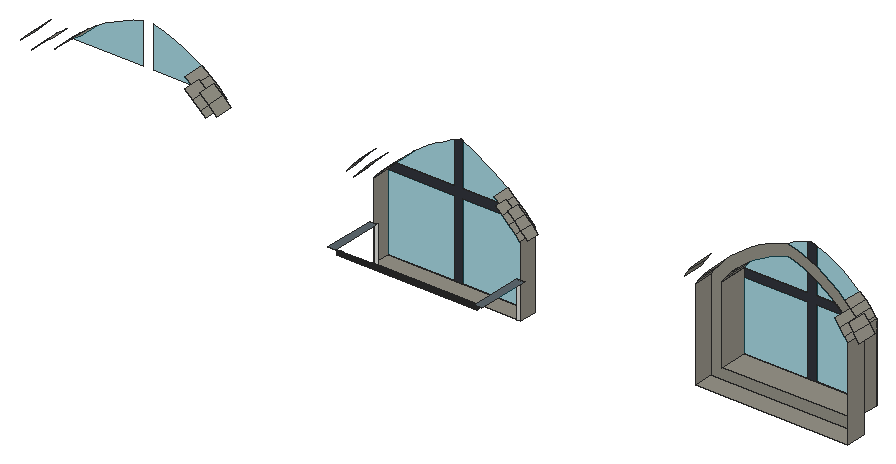
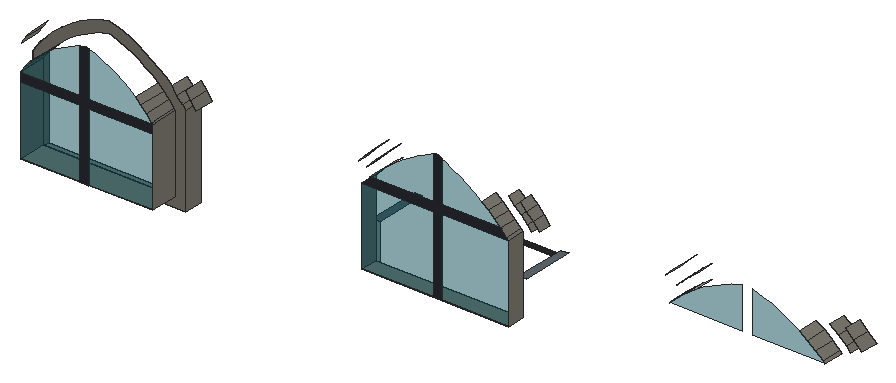
# SketchUp Ruby script. Lengths in inches.
U = 1.inch
M = Sketchup.active_model
def pt(a) = Geom::Point3d.new(a.map { |v| v * U })
def face(e, loops, mat)
  f = e.add_face(loops[0].map { |a| pt(a) })
  loops[1..].each { |l| e.add_face(l.map { |a| pt(a) }).erase! }
  f.material = f.back_material = mat if mat
  f
end
# faces: each face lists its corners as indices into pts; further lists are holes
def faces(e, pts, list, mat = nil) = list.each { |f| face(e, (f[0].is_a?(Array) ? f : [f]).map { |l| l.map { |i| pts[i] } }, mat) }
# xy, xz, yz: faces in a plane at the given z, y or x. An outline is a flat list of corners, or four numbers for a rectangle; further outlines are holes
def ring(l) = l.size == 4 ? [[l[0], l[1]], [l[2], l[1]], [l[2], l[3]], [l[0], l[3]]] : l.each_slice(2).to_a
def flat(e, list, mat, &to3) = list.each { |f| face(e, (f[0].is_a?(Array) ? f : [f]).map { |l| ring(l).map { |u, v| to3.(u, v) } }, mat) }
def xy(e, z, list, mat = nil) = flat(e, list, mat) { |x, y| [x, y, z] }
def xz(e, y, list, mat = nil) = flat(e, list, mat) { |x, z| [x, y, z] }
def yz(e, x, list, mat = nil) = flat(e, list, mat) { |y, z| [x, y, z] }
def lines(e, pts, list) = list.each { |a, b| e.add_line(pt(pts[a]), pt(pts[b])) }
# prism: a flat outline (further loops are holes) pulled along v
def prism(e, loops, v, mat = nil)
  f = face(e, loops, mat); d = Geom::Vector3d.new(v.map { |x| x * U })
  f.pushpull(f.normal.samedirection?(d) ? d.length : -d.length)
end
def box(e, o, s, mat = nil) = prism(e, [[o, [o[0] + s[0], o[1], o[2]], [o[0] + s[0], o[1] + s[1], o[2]], [o[0], o[1] + s[1], o[2]]]], [0, 0, s[2]], mat)
def at(x, y, z, deg = 0) = Geom::Transformation.translation(pt([x, y, z])) * Geom::Transformation.rotation(ORIGIN, Z_AXIS, deg.degrees)
def axes(o, x, y, z) = Geom::Transformation.new([*x, 0, *y, 0, *z, 0, *pt(o).to_a, 1])
def part(name) = M.definitions.add(name)
# library, detail: a bought-in or finely detailed component or shape, given as its bounding box
def library(name, o, s) = part(name).tap { |d| box(d.entities, o, s) }
def detail(e, o, s) = box(e.add_group.entities, o, s)
def put(e, d, t, mat = nil) = e.add_instance(d, t).tap { |i| i.material = mat if mat }
def group(e, t, mat = nil) = e.add_group.tap { |g| g.transformation = t; g.material = mat if mat }.entities
root = M.entities
M.materials.add("[Color M07]").color = [58, 58, 58]
M.materials.add("[Formica Graystone]").color = [149, 146, 135]
M.materials.add("[Formica Laminate Dark]").color = [50, 53, 60]
M.materials.add("[Formica Speckled Grey]").color = [94, 105, 111]
M.materials.add("[Translucent Glass Tinted]").color = [4, 106, 127]
M.materials["[Translucent Glass Tinted]"].alpha = 0.48
xy(root,454.81,[[376.06,148.68,450.98,158.3]],"[Formica Graystone]")
xy(root,456.09,[[222.16,144.04,294.2,152.54]],"[Formica Graystone]")
xy(root,459.9,[[381.16,158.3,445.88,172.24]],"[Formica Graystone]")
xy(root,471.52,[[287.21,119.22,287.43,119.22,287.63,119.28,287.8125,119.39,287.96,119.54,288.07,119.72,288.12,119.93,288.12,120.14,288.06,120.35,287.95,120.53,287.8,120.68,287.61,120.78,287.41,120.83,287.2,120.83,286.99,120.77,286.81,120.67,286.66,120.51,286.56,120.33,286.5,120.125,286.51,119.91,286.5625,119.71,286.67,119.52,286.82,119.375,287.01,119.27]])
xy(root,471.61,[[269.03,119.22,269.24,119.22,269.44,119.28,269.625,119.39,269.77,119.54,269.88,119.72,269.93,119.93,269.93,120.14,269.87,120.35,269.76,120.53,269.67,120.62,268.58,120.62,268.47,120.51,268.37,120.33,268.32,120.125,268.32,119.91,268.375,119.71,268.48,119.52,268.64,119.375,268.82,119.27],[268.58,120.62,269.67,120.62,269.61,120.68,269.43,120.78,269.22,120.83,269.01,120.83,268.8,120.77,268.62,120.67]])
xy(root,471.82,[[251.53,119.22,251.74,119.22,251.94,119.28,252.125,119.39,252.27,119.54,252.38,119.72,252.43,119.93,252.43,120.14,252.37,120.35,252.26,120.53,252.11,120.68,252.06,120.71,251.19,120.71,251.12,120.67,250.97,120.51,250.87,120.33,250.82,120.125,250.82,119.91,250.875,119.71,250.98,119.52,251.14,119.375,251.32,119.27],[254.4,119.22,254.61,119.22,254.82,119.28,255,119.39,255.15,119.54,255.25,119.72,255.31,119.93,255.3,120.14,255.25,120.35,255.14,120.53,254.99,120.68,254.93,120.71,254.07,120.71,254,120.67,253.85,120.51,253.75,120.33,253.69,120.125,253.69,119.91,253.75,119.71,253.86,119.52,254.01,119.375,254.2,119.27],[257.53,119.22,257.74,119.22,257.94,119.28,258.125,119.39,258.27,119.54,258.38,119.72,258.43,119.93,258.43,120.14,258.37,120.35,258.26,120.53,258.11,120.68,258.06,120.71,257.19,120.71,257.12,120.67,256.97,120.51,256.87,120.33,256.82,120.125,256.82,119.91,256.875,119.71,256.98,119.52,257.14,119.375,257.32,119.27],[266.15,119.22,266.36,119.22,266.57,119.28,266.75,119.39,266.9,119.54,267,119.72,267.06,119.93,267.05,120.14,267,120.35,266.89,120.53,266.74,120.68,266.68,120.71,265.82,120.71,265.75,120.67,265.6,120.51,265.5,120.33,265.44,120.125,265.44,119.91,265.5,119.71,265.61,119.52,265.76,119.375,265.95,119.27],[251.19,120.71,252.06,120.71,251.93,120.78,251.72,120.83,251.51,120.83,251.3,120.77],
  [254.07,120.71,254.93,120.71,254.8,120.78,254.6,120.83,254.38,120.83,254.18,120.77],[257.19,120.71,258.06,120.71,257.93,120.78,257.72,120.83,257.51,120.83,257.3,120.77],[265.82,120.71,266.68,120.71,266.55,120.78,266.35,120.83,266.13,120.83,265.93,120.77]])
xy(root,471.83,[[274.78,119.22,274.99,119.22,275.19,119.28,275.375,119.39,275.52,119.54,275.63,119.72,275.68,119.93,275.68,120.14,275.62,120.35,275.51,120.53,275.36,120.68,275.18,120.78,274.97,120.83,274.76,120.83,274.55,120.77,274.37,120.67,274.22,120.51,274.12,120.33,274.07,120.125,274.07,119.91,274.125,119.71,274.23,119.52,274.39,119.375,274.57,119.27]])
xy(root,472.05,[[231.4,119.22,231.61,119.22,231.82,119.28,232,119.39,232.15,119.54,232.25,119.72,232.31,119.93,232.3,120.14,232.25,120.35,232.14,120.53,231.99,120.68,231.88,120.74,231.12,120.74,231,120.67,230.85,120.51,230.75,120.33,230.69,120.125,230.69,119.91,230.75,119.71,230.86,119.52,231.01,119.375,231.2,119.27],[237.15,119.22,237.36,119.22,237.57,119.28,237.75,119.39,237.9,119.54,238,119.72,238.06,119.93,238.05,120.14,238,120.35,237.89,120.53,237.74,120.68,237.63,120.74,236.87,120.74,236.75,120.67,236.6,120.51,236.5,120.33,236.44,120.125,236.44,119.91,236.5,119.71,236.61,119.52,236.76,119.375,236.95,119.27],[248.65,119.22,248.86,119.22,249.07,119.28,249.25,119.39,249.4,119.54,249.5,119.72,249.56,119.93,249.55,120.14,249.5,120.35,249.39,120.53,249.24,120.68,249.13,120.74,248.37,120.74,248.25,120.67,248.1,120.51,248,120.33,247.94,120.125,247.94,119.91,248,119.71,248.11,119.52,248.26,119.375,248.45,119.27],[271.9,119.22,272.11,119.22,272.32,119.28,272.5,119.39,272.65,119.54,272.75,119.72,272.81,119.93,272.8,120.14,272.75,120.35,272.64,120.53,272.49,120.68,272.38,120.74,271.62,120.74,271.5,120.67,271.35,120.51,271.25,120.33,271.19,120.125,271.19,119.91,271.25,119.71,271.36,119.52,271.51,119.375,271.7,119.27],[290.78,119.22,290.99,119.22,291.19,119.28,291.375,119.39,291.52,119.54,291.63,119.72,291.68,119.93,291.68,120.14,291.62,120.35,291.51,120.53,291.36,120.68,291.25,120.74,290.49,120.74,290.37,120.67,290.22,120.51,290.12,120.33,290.07,120.125,290.07,119.91,290.125,119.71,290.23,119.52,290.39,119.375,290.57,119.27],
  [231.12,120.74,231.88,120.74,231.8,120.78,231.6,120.83,231.38,120.83,231.18,120.77],[236.87,120.74,237.63,120.74,237.55,120.78,237.35,120.83,237.13,120.83,236.93,120.77],[248.37,120.74,249.13,120.74,249.05,120.78,248.85,120.83,248.63,120.83,248.43,120.77],[271.62,120.74,272.38,120.74,272.3,120.78,272.1,120.83,271.88,120.83,271.68,120.77],[290.49,120.74,291.25,120.74,291.18,120.78,290.97,120.83,290.76,120.83,290.55,120.77]])
xy(root,472.27,[[225.65,119.22,225.86,119.22,226.07,119.28,226.25,119.39,226.4,119.54,226.5,119.72,226.56,119.93,226.55,120.14,226.5,120.35,226.39,120.53,226.24,120.68,226.18,120.71,225.32,120.71,225.25,120.67,225.1,120.51,225,120.33,224.94,120.125,224.94,119.91,225,119.71,225.11,119.52,225.26,119.375,225.45,119.27],[228.53,119.22,228.74,119.22,228.94,119.28,229.125,119.39,229.27,119.54,229.38,119.72,229.43,119.93,229.43,120.14,229.37,120.35,229.26,120.53,229.11,120.68,229.06,120.71,228.19,120.71,228.12,120.67,227.97,120.51,227.87,120.33,227.82,120.125,227.82,119.91,227.875,119.71,227.98,119.52,228.14,119.375,228.32,119.27],[234.28,119.22,234.49,119.22,234.69,119.28,234.875,119.39,235.02,119.54,235.13,119.72,235.18,119.93,235.18,120.14,235.12,120.35,235.01,120.53,234.86,120.68,234.81,120.71,233.94,120.71,233.87,120.67,233.72,120.51,233.62,120.33,233.57,120.125,233.57,119.91,233.625,119.71,233.73,119.52,233.89,119.375,234.07,119.27],[242.9,119.22,243.11,119.22,243.32,119.28,243.5,119.39,243.65,119.54,243.75,119.72,243.81,119.93,243.8,120.14,243.75,120.35,243.64,120.53,243.49,120.68,243.43,120.71,242.57,120.71,242.5,120.67,242.35,120.51,242.25,120.33,242.19,120.125,242.19,119.91,242.25,119.71,242.36,119.52,242.51,119.375,242.7,119.27],[260.4,119.22,260.61,119.22,260.82,119.28,261,119.39,261.15,119.54,261.25,119.72,261.31,119.93,261.3,120.14,261.25,120.35,261.14,120.53,260.99,120.68,260.93,120.71,260.07,120.71,260,120.67,259.85,120.51,259.75,120.33,259.69,120.125,259.69,119.91,259.75,119.71,259.86,119.52,260.01,119.375,260.2,119.27],
  [283.53,119.22,283.74,119.22,283.94,119.28,284.125,119.39,284.27,119.54,284.38,119.72,284.43,119.93,284.43,120.14,284.37,120.35,284.26,120.53,284.11,120.68,284.06,120.71,283.19,120.71,283.12,120.67,282.97,120.51,282.87,120.33,282.82,120.125,282.82,119.91,282.875,119.71,282.98,119.52,283.14,119.375,283.32,119.27],[225.32,120.71,226.18,120.71,226.05,120.78,225.85,120.83,225.63,120.83,225.43,120.77],[228.19,120.71,229.06,120.71,228.93,120.78,228.72,120.83,228.51,120.83,228.3,120.77],[233.94,120.71,234.81,120.71,234.68,120.78,234.47,120.83,234.26,120.83,234.05,120.77],[242.57,120.71,243.43,120.71,243.3,120.78,243.1,120.83,242.88,120.83,242.68,120.77],
  [260.07,120.71,260.93,120.71,260.8,120.78,260.6,120.83,260.38,120.83,260.18,120.77],[283.19,120.71,284.06,120.71,283.93,120.78,283.72,120.83,283.51,120.83,283.3,120.77]])
xy(root,472.48,[[240.03,119.22,240.24,119.22,240.44,119.28,240.625,119.39,240.77,119.54,240.88,119.72,240.93,119.93,240.93,120.14,240.87,120.35,240.76,120.53,240.67,120.62,239.58,120.62,239.47,120.51,239.37,120.33,239.32,120.125,239.32,119.91,239.375,119.71,239.48,119.52,239.64,119.375,239.82,119.27],[245.78,119.22,245.99,119.22,246.19,119.28,246.375,119.39,246.52,119.54,246.63,119.72,246.68,119.93,246.68,120.14,246.62,120.35,246.51,120.53,246.42,120.62,245.33,120.62,245.22,120.51,245.12,120.33,245.07,120.125,245.07,119.91,245.125,119.71,245.23,119.52,245.39,119.375,245.57,119.27],[263.28,119.22,263.49,119.22,263.69,119.28,263.875,119.39,264.02,119.54,264.13,119.72,264.18,119.93,264.18,120.14,264.12,120.35,264.01,120.53,263.92,120.62,262.83,120.62,262.72,120.51,262.62,120.33,262.57,120.125,262.57,119.91,262.625,119.71,262.73,119.52,262.89,119.375,263.07,119.27],[277.65,119.22,277.86,119.22,278.07,119.28,278.25,119.39,278.4,119.54,278.5,119.72,278.56,119.93,278.55,120.14,278.5,120.35,278.39,120.53,278.29,120.62,277.2,120.62,277.1,120.51,277,120.33,276.94,120.125,276.94,119.91,277,119.71,277.11,119.52,277.26,119.375,277.45,119.27],[280.53,119.22,280.74,119.22,280.94,119.28,281.125,119.39,281.27,119.54,281.38,119.72,281.43,119.93,281.43,120.14,281.37,120.35,281.26,120.53,281.17,120.62,280.08,120.62,279.97,120.51,279.87,120.33,279.82,120.125,279.82,119.91,279.875,119.71,279.98,119.52,280.14,119.375,280.32,119.27],
  [239.58,120.62,240.67,120.62,240.61,120.68,240.43,120.78,240.22,120.83,240.01,120.83,239.8,120.77,239.62,120.67],[245.33,120.62,246.42,120.62,246.36,120.68,246.18,120.78,245.97,120.83,245.76,120.83,245.55,120.77,245.37,120.67],[262.83,120.62,263.92,120.62,263.86,120.68,263.68,120.78,263.47,120.83,263.26,120.83,263.05,120.77,262.87,120.67],[277.2,120.62,278.29,120.62,278.24,120.68,278.05,120.78,277.85,120.83,277.63,120.83,277.43,120.77,277.25,120.67],[280.08,120.62,281.17,120.62,281.11,120.68,280.93,120.78,280.72,120.83,280.51,120.83,280.3,120.77,280.12,120.67]])
xy(root,473.83,[[220.36,118.22,223.91,144.04],[292.38,118.22,295.93,144.04]],"[Formica Speckled Grey]")
xz(root,144.04,[[222.16,456.09,223.91,473.83],[292.38,456.09,294.2,473.83]])
xz(root,152.54,[[255.17,456.09,258.8125,456.09,258.8125,493.75,294.1,493.75,293.375,494.56,290.42,497.6,290.14,497.87,258.8125,497.87,258.8125,519.11,258.07,519.42,257.1,519.04,255.17,518.1875,255.17,497.87,225.91,497.87,223.04,494.78,222.16,493.75,255.17,493.75]],"[Formica Laminate Dark]")
xz(root,152.54,[[222.16,456.09,255.17,493.75],[258.8125,456.09,294.2,456.09,294.2,493.63,294.1,493.75,258.8125,493.75],[225.91,497.87,255.17,497.87,255.17,518.1875,253.24,517.33,249.47,515.46,245.78,513.41,242.1875,511.2,238.7,508.83,235.32,506.31,232.06,503.64,228.92,500.82],[258.8125,497.87,290.14,497.87,287.34,500.53,284.15,503.33,280.85,505.99,277.45,508.52,273.94,510.92,270.34,513.16,266.65,515.27,262.89,517.22,260.125,518.51,259.04,519.01,258.8125,519.11]],"[Translucent Glass Tinted]")
xz(root,154.22,[[65.73,495.36,101.05,495.36,101.05,515.6875,96.28,514.21,91.6,512.45,87.04,510.4,82.61,508.07,78.34,505.48,74.23,502.63,70.3,499.54,66.57,496.21],[105.93,495.36,142.02,495.36,142.02,495.45,141.16,496.32,137.45,499.65,133.54,502.75,129.4375,505.6,125.17,508.18,120.74,510.5,116.18,512.53,111.5,514.27,106.73,515.71,105.93,515.9]],"[Translucent Glass Tinted]")
xz(root,158.3,[[[376.06,454.81,450.98,454.81,450.98,499.35,449.48,501.6,446.98,504.875,444.25,507.97,441.33,510.88,438.22,513.58,434.93,516.07,431.48,518.33,427.89,520.36,424.17,522.13,420.34,523.66,417.87,524.45,416.41,524.92,413.6,525.62,410.81,524.83,409.22,524.28,406.91,523.47,403.1,521.87,399.4,520.04,395.8125,517.98,392.36,515.7,389.0625,513.22,385.92,510.53,382.95,507.66,380.16,504.61,377.57,501.39,376.06,499.26],[381.16,459.9,381.16,497.63,381.64,498.3125,384.03,501.28,386.61,504.1,389.35,506.76,392.25,509.24,395.3,511.53,398.49,513.64,401.8,515.54,405.22,517.23,408.74,518.71,412.35,519.97,413.68,520.34,415.02,520.01,418.61,518.85,422.13,517.46,425.54,515.83,428.83,513.97,431.99,511.9,435,509.62,437.86,507.14,440.54,504.48,443.03,501.64,445.33,498.64,445.88,497.81,445.88,459.9]]],"[Formica Graystone]")
xz(root,172.24,[[412.35,459.9,416.87,459.9,416.87,493.68,445.88,493.68,445.88,497.63,416.87,497.63,416.87,519.42,415.02,520.01,413.68,520.34,412.35,519.97,412.35,497.63,381.16,497.63,381.16,493.68,412.35,493.68]],"[Formica Laminate Dark]")
xz(root,172.24,[[381.16,459.9,412.35,493.68],[416.87,459.9,445.88,493.68],[381.16,497.63,412.35,497.63,412.35,519.97,408.74,518.71,405.22,517.23,401.8,515.54,398.49,513.64,395.3,511.53,392.25,509.24,389.35,506.76,386.61,504.1,384.03,501.28,381.64,498.3125],[416.87,497.63,445.88,497.63,445.88,497.81,445.33,498.64,443.03,501.64,440.54,504.48,437.86,507.14,435,509.62,431.99,511.9,428.83,513.97,425.54,515.83,422.13,517.46,418.61,518.85,416.87,519.42]],"[Translucent Glass Tinted]")
yz(root,222.16,[[144.04,456.09,152.54,493.75]],"[Formica Graystone]")
yz(root,223.91,[[119.86,471.17,119.64,471.2,119.42,471.29,119.24,471.43,119.1,471.61,119.02,471.82,118.99,472.05,119.02,472.27,119.1,472.48,119.24,472.67,119.42,472.81,119.64,472.89,119.86,472.92,120.09,472.89,120.3,472.81,120.48,472.67,120.62,472.48,120.71,472.27,120.74,472.05,120.71,471.82,120.62,471.61,120.48,471.43,120.3,471.29,120.09,471.2]])
yz(root,294.2,[[144.04,456.09,152.54,493.63]],"[Formica Graystone]")
yz(root,376.06,[[148.68,454.81,158.3,499.26]],"[Formica Graystone]")
yz(root,381.16,[[158.3,459.9,172.24,497.63]],"[Formica Graystone]")
yz(root,445.88,[[158.3,459.9,172.24,497.81]],"[Formica Graystone]")
yz(root,450.98,[[148.68,454.81,158.3,499.35]],"[Formica Graystone]")
p = [[223.91,119.42,471.29],[223.91,119.64,471.2],[292.38,119.64,471.2],[292.38,119.42,471.29],[223.91,119.86,471.17],[292.38,119.86,471.17],
  [223.91,120.09,471.2],[292.38,120.09,471.2],[223.91,120.3,471.29],[292.38,120.3,471.29],[223.91,119.24,471.43],[292.38,119.24,471.43],
  [223.91,120.48,471.43],[292.38,120.48,471.43],[223.91,119.1,471.61],[292.38,119.1,471.61],[223.91,120.62,471.61],[268.58,120.62,471.61],
  [269.67,120.62,471.61],[292.38,120.62,471.61],[223.91,119.02,471.82],[292.38,119.02,471.82],[223.91,120.71,471.82],[251.19,120.71,471.82],
  [252.06,120.71,471.82],[254.07,120.71,471.82],[254.93,120.71,471.82],[257.19,120.71,471.82],[258.06,120.71,471.82],[265.82,120.71,471.82],
  [266.68,120.71,471.82],[292.38,120.71,471.82],[223.91,118.99,472.05],[292.38,118.99,472.05],[223.91,120.74,472.05],[231.12,120.74,472.05],
  [231.88,120.74,472.05],[236.87,120.74,472.05],[237.63,120.74,472.05],[248.37,120.74,472.05],[249.13,120.74,472.05],[271.62,120.74,472.05],
  [272.38,120.74,472.05],[290.49,120.74,472.05],[291.25,120.74,472.05],[292.38,120.74,472.05],[223.91,119.02,472.27],[292.38,119.02,472.27],
  [223.91,120.71,472.27],[225.32,120.71,472.27],[226.18,120.71,472.27],[228.19,120.71,472.27],[229.06,120.71,472.27],[233.94,120.71,472.27],
  [234.81,120.71,472.27],[242.57,120.71,472.27],[243.43,120.71,472.27],[260.07,120.71,472.27],[260.93,120.71,472.27],[283.19,120.71,472.27],
  [284.06,120.71,472.27],[292.38,120.71,472.27],[223.91,119.1,472.48],[292.38,119.1,472.48],[223.91,120.62,472.48],[239.58,120.62,472.48],
  [240.67,120.62,472.48],[245.33,120.62,472.48],[246.42,120.62,472.48],[262.83,120.62,472.48],[263.92,120.62,472.48],[277.2,120.62,472.48],
  [278.29,120.62,472.48],[280.08,120.62,472.48],[281.17,120.62,472.48],[292.38,120.62,472.48],[223.91,119.24,472.67],[292.38,119.24,472.67],
  [223.91,120.48,472.67],[292.38,120.48,472.67],[223.91,119.42,472.81],[292.38,119.42,472.81],[223.91,120.3,472.81],[292.38,120.3,472.81],
  [223.91,119.64,472.89],[292.38,119.64,472.89],[223.91,120.09,472.89],[292.38,120.09,472.89],[223.91,119.86,472.92],[292.38,119.86,472.92],
  [294.2,144.04,493.63],[293.375,144.04,494.56],[293.375,152.54,494.56],[294.1,152.54,493.75],[294.2,152.54,493.63],[223.04,144.04,494.78],
  [222.16,144.04,493.75],[222.16,152.54,493.75],[223.04,152.54,494.78],[290.42,144.04,497.6],[290.42,152.54,497.6],[225.91,144.04,497.87],
  [225.91,152.54,497.87],[217.65,144.04,495.41],[219.67,144.04,497.78],[219.67,137.66,497.78],[217.65,137.66,495.41],[296.67,144.04,497.63],
  [298.71,144.04,495.36],[298.71,137.66,495.36],[296.67,137.66,497.63],[66.57,144.04,496.21],[65.73,144.04,495.36],[65.73,154.22,495.36],
  [66.57,154.22,496.21],[142.02,144.04,495.45],[141.16,144.04,496.32],[141.16,154.22,496.32],[142.02,154.22,495.45],[70.3,144.04,499.54],
  [70.3,154.22,499.54],[137.45,144.04,499.65],[137.45,154.22,499.65],[216.84,144.04,500.3],[213.87,144.04,496.8],[213.87,137.66,496.8],
  [216.84,137.66,500.3],[302.49,144.04,496.8],[299.44,144.04,500.21],[299.44,137.66,500.21],[302.49,137.66,496.8],[61.3,144.04,497.1875],
  [63.52,144.04,499.43],[63.52,135.41,499.43],[61.3,135.41,497.1875],[144.23,144.04,499.52],[146.45,144.04,497.26],[146.45,135.41,497.26],
  [144.23,135.41,499.52],[293.59,144.04,500.81],[293.59,137.66,500.81],[287.34,144.04,500.53],[287.34,152.54,500.53],[290.14,152.54,497.87],
  [381.64,158.3,498.3125],[381.16,158.3,497.63],[381.16,172.24,497.63],[381.64,172.24,498.3125],[222.68,144.04,501.01],[222.68,137.66,501.01],
  [445.88,158.3,497.81],[445.33,158.3,498.64],[445.33,172.24,498.64],[445.88,172.24,497.81],[228.92,144.04,500.82],[228.92,152.54,500.82],
  [384.03,158.3,501.28],[384.03,172.24,501.28],[443.03,158.3,501.64],[443.03,172.24,501.64],[376.06,158.3,499.26],[377.57,158.3,501.39],
  [377.57,148.68,501.39],[376.06,148.68,499.26],[449.48,158.3,501.6],[450.98,158.3,499.35],[450.98,148.68,499.35],[449.48,148.68,501.6],
  [67.45,144.04,502.9375],[67.45,135.41,502.9375],[59.68,144.04,503.46],[55.73,144.04,499.48],[55.73,135.41,499.48],[59.68,135.41,503.46],
  [140.32,144.04,503.05],[140.32,135.41,503.05],[152.02,144.04,499.53],[148.09,144.04,503.55],[148.09,135.41,503.55],[152.02,135.41,499.53],
  [74.23,144.04,502.63],[74.23,154.22,502.63],[133.54,144.04,502.75],[133.54,154.22,502.75],[296.25,144.04,503.5],[296.25,137.66,503.5],
  [219.97,144.04,503.65],[219.97,137.66,503.65],[284.15,144.04,503.33],[284.15,152.54,503.33],[290.38,144.04,503.86],[290.38,137.66,503.86],
  [232.06,144.04,503.64],[232.06,152.54,503.64],[373.34,158.3,504.58],[370.76,158.3,500.95],[370.76,148.68,500.95],[373.34,148.68,504.58],
  [456.27,158.3,500.95],[453.8,158.3,504.68],[453.8,148.68,504.68],[456.27,148.68,500.95],[225.83,144.04,504.11],[225.83,137.66,504.11],
  [386.61,158.3,504.1],[386.61,172.24,504.1],[380.16,158.3,504.61],[380.16,148.68,504.61],[446.98,158.3,504.875],[446.98,148.68,504.875],
  [440.54,158.3,504.48],[440.54,172.24,504.48],[78.34,144.04,505.48],[78.34,154.22,505.48],[129.4375,144.04,505.6],[129.4375,154.22,505.6],
  [71.59,144.04,506.2],[71.59,135.41,506.2],[136.18,144.04,506.32],[136.18,135.41,506.32],[280.85,144.04,505.99],[280.85,152.54,505.99],
  [63.87,144.04,507.2],[63.87,135.41,507.2],[143.91,144.04,507.3],[143.91,135.41,507.3],[292.9375,144.04,506.65],[292.9375,137.66,506.65],
  [235.32,144.04,506.31],[235.32,152.54,506.31],[223.25,144.04,506.87],[223.25,137.66,506.87],[287.06,144.04,506.78],[287.06,137.66,506.78],
  [229.125,144.04,507.06],[229.125,137.66,507.06],[389.35,158.3,506.76],[389.35,172.24,506.76],[437.86,158.3,507.14],[437.86,172.24,507.14],
  [376.14,158.3,508.06],[376.14,148.68,508.06],[382.95,158.3,507.66],[382.95,148.68,507.66],[451.07,158.3,508.24],[451.07,148.68,508.24],
  [444.25,158.3,507.97],[444.25,148.68,507.97]]
faces(root,p,[[0,1,2,3],[1,4,5,2],[4,6,7,5],[6,8,9,7],[10,0,3,11],[8,12,13,9],[14,10,11,15],[12,16,17,18,19,13],
  [20,14,15,21],[16,22,23,24,25,26,27,28,29,30,31,19,18,17],[32,20,21,33],[22,34,35,36,37,38,39,40,41,42,43,44,45,31,30,29,28,27,26,25,24,23],[46,32,33,47],[34,48,49,50,51,52,53,54,55,56,57,58,59,60,61,45,44,43,42,41,40,39,38,37,36,35],[62,46,47,63],[48,64,65,66,67,68,69,70,71,72,73,74,75,61,60,59,58,57,56,55,54,53,52,51,50,49],
  [76,62,63,77],[64,78,79,75,74,73,72,71,70,69,68,67,66,65],[80,76,77,81],[78,82,83,79],[84,80,81,85],[82,86,87,83],[88,84,85,89],[86,88,89,87]],"[Color M07]")
faces(root,p,[[90,91,92,93,94],[95,96,97,98],[91,99,100,92],[101,95,98,102],[103,104,105,106],[107,108,109,110],[111,112,113,114],[115,116,117,118],
  [119,111,114,120],[116,121,122,117],[123,124,125,126],[127,128,129,130],[131,132,133,134],[135,136,137,138],[139,107,110,140],[99,141,142,143,100],
  [144,145,146,147],[104,148,149,105],[150,151,152,153],[154,101,102,155],[156,144,147,157],[151,158,159,152],[160,161,162,163],[164,165,166,167],
  [132,168,169,133],[170,171,172,173],[174,135,138,175],[176,177,178,179],[180,119,120,181],[121,182,183,122],[128,184,185,129],[186,123,126,187],
  [141,188,189,142],[190,139,140,191],[192,154,155,193],[194,195,196,197],[198,199,200,201],[148,202,203,149],[204,156,157,205],[161,206,207,162],
  [208,164,167,209],[158,210,211,159],[212,180,181,213],[182,214,215,183],[168,216,217,169],[218,174,175,219],[188,220,221,189],[222,170,173,223],
  [177,224,225,178],[184,226,227,185],[228,192,193,229],[230,186,187,231],[232,190,191,233],[202,234,235,203],[236,204,205,237],[210,238,239,211],
  [240,194,197,241],[206,242,243,207],[199,244,245,200],[246,208,209,247]],"[Formica Graystone]")
